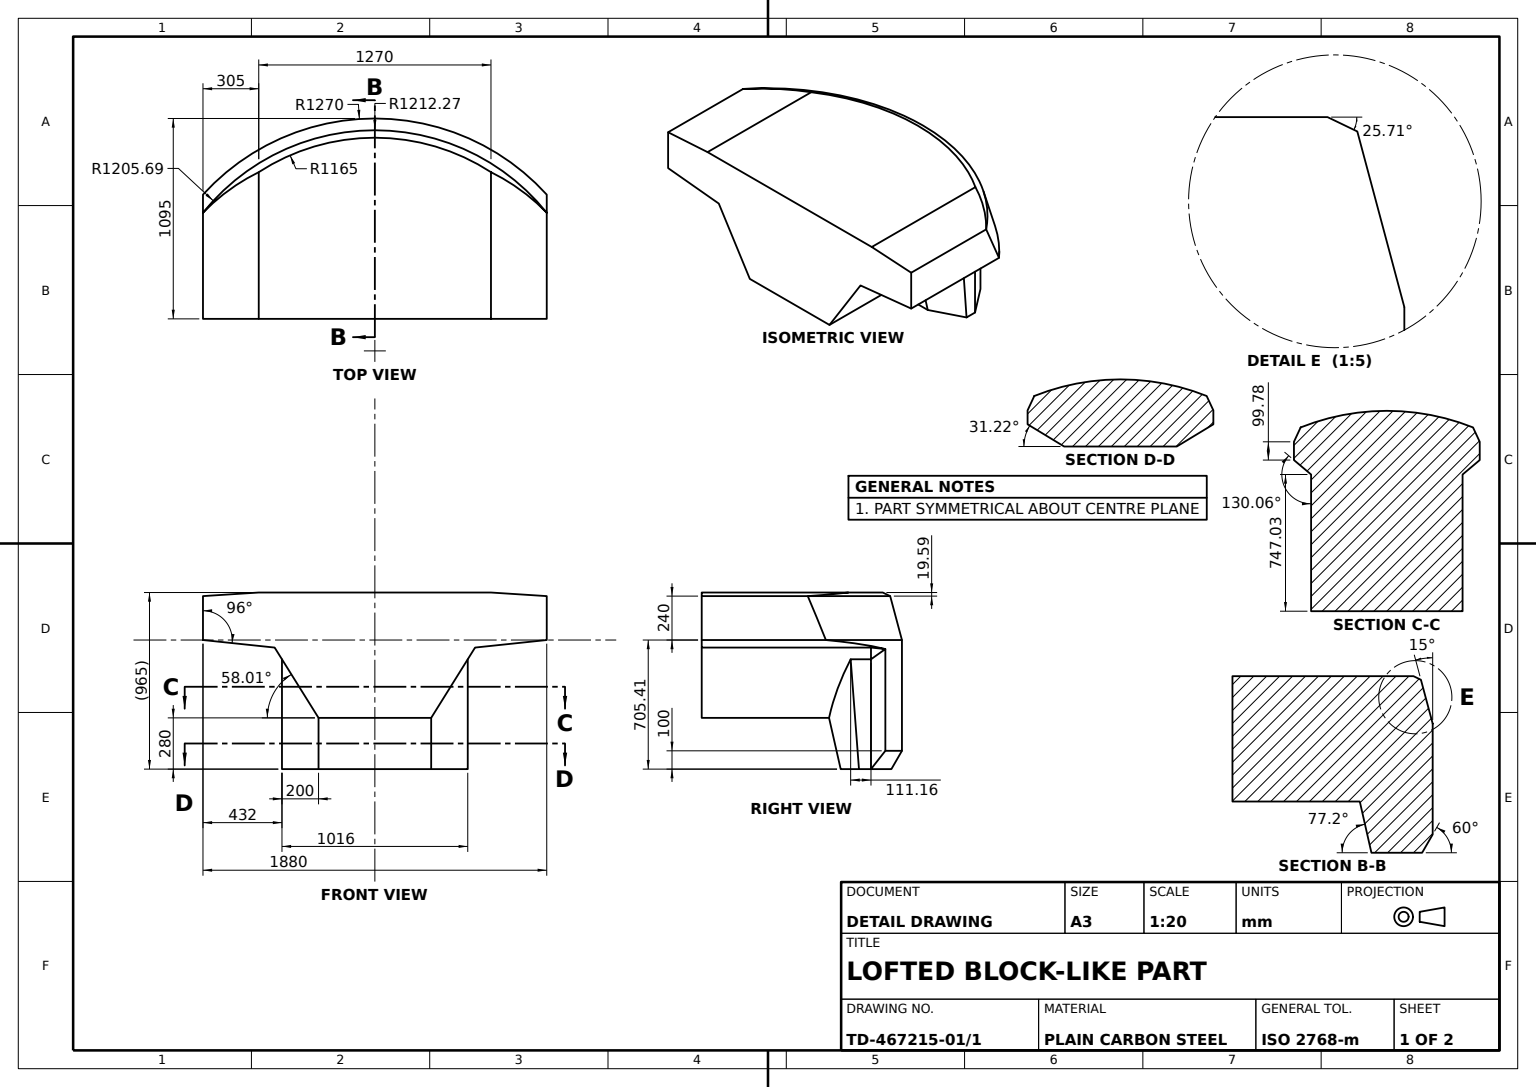
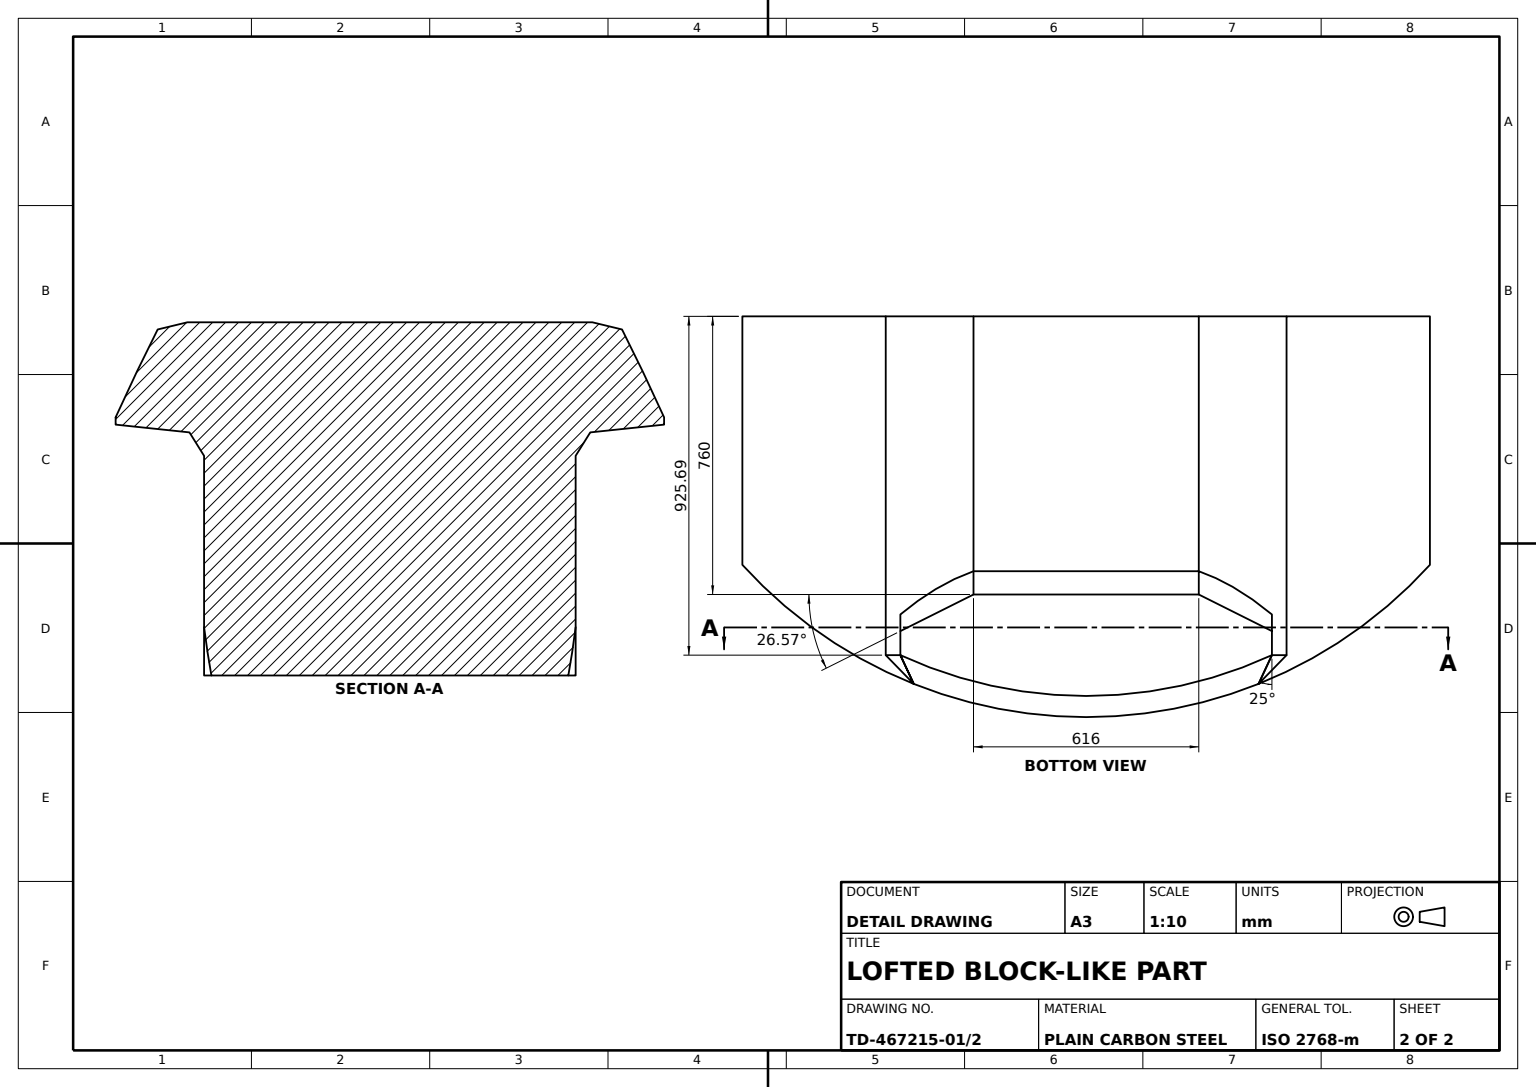
ISO-10303-21;
HEADER;
FILE_DESCRIPTION((''),'2;1');
FILE_NAME('','',(''),(''),'','','');
FILE_SCHEMA(('AUTOMOTIVE_DESIGN'));
ENDSEC;
DATA;
#1=APPLICATION_CONTEXT('');
#2=PRODUCT_CONTEXT('',#1,'mechanical');
#3=PRODUCT('','','',(#2));
#4=PRODUCT_DEFINITION_FORMATION('','',#3);
#5=PRODUCT_DEFINITION_CONTEXT('',#1,'design');
#6=PRODUCT_DEFINITION('','',#4,#5);
#7=PRODUCT_DEFINITION_SHAPE('','',#6);
#8=(LENGTH_UNIT()NAMED_UNIT(*)SI_UNIT(.MILLI.,.METRE.));
#9=(NAMED_UNIT(*)PLANE_ANGLE_UNIT()SI_UNIT($,.RADIAN.));
#10=(NAMED_UNIT(*)SI_UNIT($,.STERADIAN.)SOLID_ANGLE_UNIT());
#11=UNCERTAINTY_MEASURE_WITH_UNIT(LENGTH_MEASURE(1.E-05),#8,'distance_accuracy_value','');
#12=(GEOMETRIC_REPRESENTATION_CONTEXT(3)GLOBAL_UNCERTAINTY_ASSIGNED_CONTEXT((#11))GLOBAL_UNIT_ASSIGNED_CONTEXT((#8,#9,#10))REPRESENTATION_CONTEXT('',''));
#13=CARTESIAN_POINT('',(-471.347784,656.147697,-1004.292698));
#14=VERTEX_POINT('',#13);
#15=CARTESIAN_POINT('',(-548.,664.204169,-925.691767));
#16=VERTEX_POINT('',#15);
#17=DIRECTION('',(-0.696304067,0.073184506,0.714006075));
#18=VECTOR('',#17,1000.);
#19=LINE('',#13,#18);
#20=EDGE_CURVE('',#14,#16,#19,.T.);
#21=ORIENTED_EDGE('',*,*,#20,.F.);
#22=CARTESIAN_POINT('',(-508.,600.170141,-925.691767));
#23=VERTEX_POINT('',#22);
#24=DIRECTION('',(-0.355078158,-0.542297561,0.761467568));
#25=VECTOR('',#24,1000.);
#26=LINE('',#13,#25);
#27=EDGE_CURVE('',#14,#23,#26,.T.);
#28=ORIENTED_EDGE('',*,*,#27,.T.);
#29=DIRECTION('',(0.529796363,-0.848124881,0.));
#30=VECTOR('',#29,1000.);
#31=LINE('',#15,#30);
#32=EDGE_CURVE('',#16,#23,#31,.T.);
#33=ORIENTED_EDGE('',*,*,#32,.F.);
#34=EDGE_LOOP('',(#21,#28,#33));
#35=FACE_OUTER_BOUND('',#34,.T.);
#36=CARTESIAN_POINT('',(-439.803143,-274.730892,-400.739829));
#37=DIRECTION('',(-0.671086691,-0.419206294,-0.611480773));
#38=DIRECTION('',(-0.67351782,0.,0.739170985));
#39=AXIS2_PLACEMENT_3D('',#36,#37,#38);
#40=PLANE('',#39);
#41=ADVANCED_FACE('',(#35),#40,.T.);
#42=CARTESIAN_POINT('',(0.,945.40503,-1030.692194));
#43=VERTEX_POINT('',#42);
#44=CARTESIAN_POINT('',(940.,945.40503,-580.045473));
#45=VERTEX_POINT('',#44);
#46=CARTESIAN_POINT('',(0.,945.40503,175.));
#47=DIRECTION('',(0.,-1.,0.));
#48=DIRECTION('',(0.,0.,-1.));
#49=AXIS2_PLACEMENT_3D('',#46,#47,#48);
#50=CIRCLE('',#49,1205.692194);
#51=EDGE_CURVE('',#43,#45,#50,.T.);
#52=ORIENTED_EDGE('',*,*,#51,.T.);
#53=CARTESIAN_POINT('',(940.,705.40503,-678.990632));
#54=VERTEX_POINT('',#53);
#55=CARTESIAN_POINT('',(940.,745.612267,-662.96898));
#56=CARTESIAN_POINT('',(940.,785.727052,-646.738003));
#57=CARTESIAN_POINT('',(940.,865.739298,-613.78401));
#58=CARTESIAN_POINT('',(940.,905.636865,-597.061233));
#59=B_SPLINE_CURVE_WITH_KNOTS('',3,(#53,#55,#56,#57,#58,#44),.UNSPECIFIED.,.F.,.F.,(4,2,4),(0.754872471,0.884630392,1.014388313),.UNSPECIFIED.);
#60=EDGE_CURVE('',#54,#45,#59,.T.);
#61=ORIENTED_EDGE('',*,*,#60,.F.);
#62=CARTESIAN_POINT('',(0.,705.40503,-1095.));
#63=VERTEX_POINT('',#62);
#64=CARTESIAN_POINT('',(0.,705.40503,175.));
#65=AXIS2_PLACEMENT_3D('',#64,#47,#48);
#66=CIRCLE('',#65,1270.);
#67=EDGE_CURVE('',#63,#54,#66,.T.);
#68=ORIENTED_EDGE('',*,*,#67,.F.);
#69=DIRECTION('',(0.,-0.965925826,-0.258819045));
#70=VECTOR('',#69,1000.);
#71=LINE('',#42,#70);
#72=EDGE_CURVE('',#43,#63,#71,.T.);
#73=ORIENTED_EDGE('',*,*,#72,.F.);
#74=EDGE_LOOP('',(#52,#61,#68,#73));
#75=FACE_OUTER_BOUND('',#74,.T.);
#76=CONICAL_SURFACE('',#49,1205.692193817,0.261799388);
#77=ADVANCED_FACE('',(#75),#76,.T.);
#78=CARTESIAN_POINT('',(508.,600.170141,-925.691767));
#79=VERTEX_POINT('',#78);
#80=CARTESIAN_POINT('',(508.,0.,-925.691767));
#81=VERTEX_POINT('',#80);
#82=CARTESIAN_POINT('',(508.,745.039237,-925.691767));
#83=VECTOR('',#47,1000.);
#84=LINE('',#82,#83);
#85=EDGE_CURVE('',#79,#81,#84,.T.);
#86=ORIENTED_EDGE('',*,*,#85,.T.);
#87=CARTESIAN_POINT('',(471.347784,100.,-1004.292698));
#88=VERTEX_POINT('',#87);
#89=CARTESIAN_POINT('',(483.369243,66.264561,-978.512595));
#90=CARTESIAN_POINT('',(495.570346,32.897774,-952.347245));
#91=B_SPLINE_CURVE_WITH_KNOTS('',3,(#87,#89,#90,#80),.UNSPECIFIED.,.F.,.F.,(4,4),(0.000000262,0.132369032),.UNSPECIFIED.);
#92=EDGE_CURVE('',#88,#81,#91,.T.);
#93=ORIENTED_EDGE('',*,*,#92,.F.);
#94=CARTESIAN_POINT('',(471.347784,656.147697,-1004.292698));
#95=VERTEX_POINT('',#94);
#96=CARTESIAN_POINT('',(471.347784,745.039237,-1004.292698));
#97=LINE('',#96,#83);
#98=EDGE_CURVE('',#95,#88,#97,.T.);
#99=ORIENTED_EDGE('',*,*,#98,.F.);
#100=DIRECTION('',(0.355078158,-0.542297561,0.761467568));
#101=VECTOR('',#100,1000.);
#102=LINE('',#94,#101);
#103=EDGE_CURVE('',#95,#79,#102,.T.);
#104=ORIENTED_EDGE('',*,*,#103,.T.);
#105=EDGE_LOOP('',(#86,#93,#99,#104));
#106=FACE_OUTER_BOUND('',#105,.T.);
#107=DIRECTION('',(-0.906307787,0.,0.422618262));
#108=DIRECTION('',(0.422618262,0.,0.906307787));
#109=AXIS2_PLACEMENT_3D('',#82,#107,#108);
#110=PLANE('',#109);
#111=ADVANCED_FACE('',(#106),#110,.F.);
#112=CARTESIAN_POINT('',(548.,664.204169,-925.691767));
#113=VERTEX_POINT('',#112);
#114=CARTESIAN_POINT('',(548.,664.204169,0.));
#115=VERTEX_POINT('',#114);
#116=DIRECTION('',(0.,0.,1.));
#117=VECTOR('',#116,1000.);
#118=LINE('',#112,#117);
#119=EDGE_CURVE('',#113,#115,#118,.T.);
#120=ORIENTED_EDGE('',*,*,#119,.T.);
#121=CARTESIAN_POINT('',(308.,280.,0.));
#122=VERTEX_POINT('',#121);
#123=DIRECTION('',(0.529796363,0.848124881,0.));
#124=VECTOR('',#123,1000.);
#125=LINE('',#121,#124);
#126=EDGE_CURVE('',#122,#115,#125,.T.);
#127=ORIENTED_EDGE('',*,*,#126,.F.);
#128=CARTESIAN_POINT('',(308.,280.,-696.363636));
#129=VERTEX_POINT('',#128);
#130=CARTESIAN_POINT('',(308.,280.,-925.691767));
#131=LINE('',#130,#117);
#132=EDGE_CURVE('',#129,#122,#131,.T.);
#133=ORIENTED_EDGE('',*,*,#132,.F.);
#134=CARTESIAN_POINT('',(508.,600.170141,-814.532565));
#135=VERTEX_POINT('',#134);
#136=CARTESIAN_POINT('',(491.980272,574.524948,-801.181759));
#137=CARTESIAN_POINT('',(475.793634,548.612558,-788.625015));
#138=CARTESIAN_POINT('',(455.337931,515.86603,-773.98717));
#139=CARTESIAN_POINT('',(451.235664,509.298914,-771.112533));
#140=CARTESIAN_POINT('',(443.00851,496.128468,-765.470873));
#141=CARTESIAN_POINT('',(438.882887,489.523962,-762.703374));
#142=CARTESIAN_POINT('',(426.477598,469.664947,-754.56895));
#143=CARTESIAN_POINT('',(418.170441,456.366429,-749.370582));
#144=CARTESIAN_POINT('',(401.48017,429.647796,-739.435331));
#145=CARTESIAN_POINT('',(393.097056,416.227682,-734.698447));
#146=CARTESIAN_POINT('',(376.252748,389.26246,-725.699057));
#147=CARTESIAN_POINT('',(367.789964,375.714806,-721.436009));
#148=CARTESIAN_POINT('',(342.321315,334.943302,-709.396412));
#149=CARTESIAN_POINT('',(325.222915,307.571316,-702.362232));
#150=B_SPLINE_CURVE_WITH_KNOTS('',3,(#134,#136,#137,#138,#139,#140,#141,#142,#143,#144,#145,#146,#147,#148,#149,#128),.UNSPECIFIED.,.F.,.F.,(4,2,2,2,2,2,2,4),(0.,0.099089394,0.123861743,0.148634091,0.198178789,0.247723486,0.297268183,0.396357577),.UNSPECIFIED.);
#151=EDGE_CURVE('',#135,#129,#150,.T.);
#152=ORIENTED_EDGE('',*,*,#151,.F.);
#153=CARTESIAN_POINT('',(508.,600.170141,-1245.));
#154=LINE('',#153,#117);
#155=EDGE_CURVE('',#79,#135,#154,.T.);
#156=ORIENTED_EDGE('',*,*,#155,.F.);
#157=LINE('',#130,#124);
#158=EDGE_CURVE('',#79,#113,#157,.T.);
#159=ORIENTED_EDGE('',*,*,#158,.T.);
#160=EDGE_LOOP('',(#120,#127,#133,#152,#156,#159));
#161=FACE_OUTER_BOUND('',#160,.T.);
#162=DIRECTION('',(0.848124881,-0.529796363,0.));
#163=AXIS2_PLACEMENT_3D('',#130,#162,#123);
#164=PLANE('',#163);
#165=ADVANCED_FACE('',(#161),#164,.T.);
#166=ORIENTED_EDGE('',*,*,#155,.T.);
#167=CARTESIAN_POINT('',(508.,0.,-860.));
#168=VERTEX_POINT('',#167);
#169=DIRECTION('',(0.,0.997142688,0.075541113));
#170=VECTOR('',#169,1000.);
#171=LINE('',#167,#170);
#172=EDGE_CURVE('',#168,#135,#171,.T.);
#173=ORIENTED_EDGE('',*,*,#172,.F.);
#174=CARTESIAN_POINT('',(508.,0.,-1245.));
#175=LINE('',#174,#117);
#176=EDGE_CURVE('',#81,#168,#175,.T.);
#177=ORIENTED_EDGE('',*,*,#176,.F.);
#178=ORIENTED_EDGE('',*,*,#85,.F.);
#179=EDGE_LOOP('',(#166,#173,#177,#178));
#180=FACE_OUTER_BOUND('',#179,.T.);
#181=DIRECTION('',(-1.,0.,0.));
#182=AXIS2_PLACEMENT_3D('',#174,#181,#116);
#183=PLANE('',#182);
#184=ADVANCED_FACE('',(#180),#183,.F.);
#185=CARTESIAN_POINT('',(-308.,280.,-696.363636));
#186=VERTEX_POINT('',#185);
#187=CARTESIAN_POINT('',(-508.,600.170141,-814.532565));
#188=VERTEX_POINT('',#187);
#189=CARTESIAN_POINT('',(-325.223184,307.571746,-702.362325));
#190=CARTESIAN_POINT('',(-342.31947,334.940347,-709.395792));
#191=CARTESIAN_POINT('',(-363.53797,368.907998,-719.425934));
#192=CARTESIAN_POINT('',(-367.774075,375.689371,-721.493893));
#193=CARTESIAN_POINT('',(-376.231258,389.228058,-725.752355));
#194=CARTESIAN_POINT('',(-380.453182,395.986728,-727.943316));
#195=CARTESIAN_POINT('',(-393.089676,416.215868,-734.694309));
#196=CARTESIAN_POINT('',(-401.473914,429.637782,-739.431731));
#197=CARTESIAN_POINT('',(-418.164445,456.356829,-749.366888));
#198=CARTESIAN_POINT('',(-426.470737,469.653963,-754.564625));
#199=CARTESIAN_POINT('',(-443.007509,496.126866,-765.407806));
#200=CARTESIAN_POINT('',(-451.239205,509.304582,-771.054287));
#201=CARTESIAN_POINT('',(-475.791522,548.609176,-788.623275));
#202=CARTESIAN_POINT('',(-491.980008,574.524526,-801.181539));
#203=B_SPLINE_CURVE_WITH_KNOTS('',3,(#185,#189,#190,#191,#192,#193,#194,#195,#196,#197,#198,#199,#200,#201,#202,#187),.UNSPECIFIED.,.F.,.F.,(4,2,2,2,2,2,2,4),(0.,0.099073271,0.123841589,0.148609906,0.198146542,0.247683177,0.297219813,0.396293084),.UNSPECIFIED.);
#204=EDGE_CURVE('',#186,#188,#203,.T.);
#205=ORIENTED_EDGE('',*,*,#204,.T.);
#206=CARTESIAN_POINT('',(-508.,0.,-860.));
#207=VERTEX_POINT('',#206);
#208=CARTESIAN_POINT('',(-508.,330.,-835.));
#209=LINE('',#208,#170);
#210=EDGE_CURVE('',#207,#188,#209,.T.);
#211=ORIENTED_EDGE('',*,*,#210,.F.);
#212=CARTESIAN_POINT('',(-308.,0.,-760.));
#213=VERTEX_POINT('',#212);
#214=DIRECTION('',(0.894427191,0.,0.447213595));
#215=VECTOR('',#214,1000.);
#216=LINE('',#206,#215);
#217=EDGE_CURVE('',#207,#213,#216,.T.);
#218=ORIENTED_EDGE('',*,*,#217,.T.);
#219=CARTESIAN_POINT('',(-308.,330.,-685.));
#220=DIRECTION('',(0.,-0.975132856,-0.221621104));
#221=VECTOR('',#220,1000.);
#222=LINE('',#219,#221);
#223=EDGE_CURVE('',#186,#213,#222,.T.);
#224=ORIENTED_EDGE('',*,*,#223,.F.);
#225=EDGE_LOOP('',(#205,#211,#218,#224));
#226=FACE_OUTER_BOUND('',#225,.T.);
#227=CARTESIAN_POINT('',(-308.,660.,-610.));
#228=CARTESIAN_POINT('',(-341.333333,0.,-776.666667));
#229=CARTESIAN_POINT('',(-341.333333,660.,-643.333333));
#230=CARTESIAN_POINT('',(-374.666667,0.,-793.333333));
#231=CARTESIAN_POINT('',(-374.666667,660.,-676.666667));
#232=CARTESIAN_POINT('',(-441.333333,0.,-826.666667));
#233=CARTESIAN_POINT('',(-441.333333,660.,-743.333333));
#234=CARTESIAN_POINT('',(-474.666667,0.,-843.333333));
#235=CARTESIAN_POINT('',(-474.666667,660.,-776.666667));
#236=CARTESIAN_POINT('',(-508.,660.,-810.));
#237=B_SPLINE_SURFACE_WITH_KNOTS('',3,1,((#212,#227),(#228,#229),(#230,#231),(#232,#233),(#234,#235),(#206,#236)),.UNSPECIFIED.,.F.,.F.,.F.,(4,2,4),(2,2),(0.,0.5,1.),(0.,1.),.UNSPECIFIED.);
#238=ADVANCED_FACE('',(#226),#237,.F.);
#239=CARTESIAN_POINT('',(308.,0.,-760.));
#240=VERTEX_POINT('',#239);
#241=DIRECTION('',(0.894427191,0.,-0.447213595));
#242=VECTOR('',#241,1000.);
#243=LINE('',#167,#242);
#244=EDGE_CURVE('',#240,#168,#243,.T.);
#245=ORIENTED_EDGE('',*,*,#244,.T.);
#246=ORIENTED_EDGE('',*,*,#172,.T.);
#247=ORIENTED_EDGE('',*,*,#151,.T.);
#248=CARTESIAN_POINT('',(308.,330.,-685.));
#249=DIRECTION('',(0.,0.975132856,0.221621104));
#250=VECTOR('',#249,1000.);
#251=LINE('',#248,#250);
#252=EDGE_CURVE('',#240,#129,#251,.T.);
#253=ORIENTED_EDGE('',*,*,#252,.F.);
#254=EDGE_LOOP('',(#245,#246,#247,#253));
#255=FACE_OUTER_BOUND('',#254,.T.);
#256=CARTESIAN_POINT('',(508.,660.,-810.));
#257=CARTESIAN_POINT('',(474.666667,0.,-843.333333));
#258=CARTESIAN_POINT('',(474.666667,660.,-776.666667));
#259=CARTESIAN_POINT('',(441.333333,0.,-826.666667));
#260=CARTESIAN_POINT('',(441.333333,660.,-743.333333));
#261=CARTESIAN_POINT('',(374.666667,0.,-793.333333));
#262=CARTESIAN_POINT('',(374.666667,660.,-676.666667));
#263=CARTESIAN_POINT('',(341.333333,0.,-776.666667));
#264=CARTESIAN_POINT('',(341.333333,660.,-643.333333));
#265=CARTESIAN_POINT('',(308.,660.,-610.));
#266=B_SPLINE_SURFACE_WITH_KNOTS('',3,1,((#167,#256),(#257,#258),(#259,#260),(#261,#262),(#263,#264),(#239,#265)),.UNSPECIFIED.,.F.,.F.,.F.,(4,2,4),(2,2),(0.,0.5,1.),(0.,1.),.UNSPECIFIED.);
#267=ADVANCED_FACE('',(#255),#266,.F.);
#268=CARTESIAN_POINT('',(940.,945.40503,0.));
#269=VERTEX_POINT('',#268);
#270=CARTESIAN_POINT('',(940.,945.40503,-1245.));
#271=LINE('',#270,#117);
#272=EDGE_CURVE('',#45,#269,#271,.T.);
#273=ORIENTED_EDGE('',*,*,#272,.F.);
#274=CARTESIAN_POINT('',(635.,965.,-801.729236));
#275=VERTEX_POINT('',#274);
#276=CARTESIAN_POINT('',(851.792172,951.072012,-671.068148));
#277=CARTESIAN_POINT('',(749.105928,957.669173,-745.703797));
#278=(BOUNDED_CURVE()B_SPLINE_CURVE(3,(#44,#276,#277,#274),.UNSPECIFIED.,.F.,.T.)B_SPLINE_CURVE_WITH_KNOTS((4,4),(0.765207077,1.110816144),.UNSPECIFIED.)CURVE()GEOMETRIC_REPRESENTATION_ITEM()RATIONAL_B_SPLINE_CURVE((1.,0.990070943,0.990070943,1.))REPRESENTATION_ITEM(''));
#279=EDGE_CURVE('',#45,#275,#278,.T.);
#280=ORIENTED_EDGE('',*,*,#279,.T.);
#281=CARTESIAN_POINT('',(635.,965.,0.));
#282=VERTEX_POINT('',#281);
#283=CARTESIAN_POINT('',(635.,965.,-1245.));
#284=LINE('',#283,#117);
#285=EDGE_CURVE('',#275,#282,#284,.T.);
#286=ORIENTED_EDGE('',*,*,#285,.T.);
#287=DIRECTION('',(0.997942605,-0.064113625,0.));
#288=VECTOR('',#287,1000.);
#289=LINE('',#268,#288);
#290=EDGE_CURVE('',#282,#269,#289,.T.);
#291=ORIENTED_EDGE('',*,*,#290,.T.);
#292=EDGE_LOOP('',(#273,#280,#286,#291));
#293=FACE_OUTER_BOUND('',#292,.T.);
#294=DIRECTION('',(-0.064113625,-0.997942605,0.));
#295=AXIS2_PLACEMENT_3D('',#270,#294,#287);
#296=PLANE('',#295);
#297=ADVANCED_FACE('',(#293),#296,.F.);
#298=CARTESIAN_POINT('',(-1496.,0.,-760.));
#299=DIRECTION('',(1.,0.,0.));
#300=VECTOR('',#299,1000.);
#301=LINE('',#298,#300);
#302=EDGE_CURVE('',#213,#240,#301,.T.);
#303=ORIENTED_EDGE('',*,*,#302,.T.);
#304=ORIENTED_EDGE('',*,*,#252,.T.);
#305=CARTESIAN_POINT('',(-1496.,280.,-696.363636));
#306=VECTOR('',#181,1000.);
#307=LINE('',#305,#306);
#308=EDGE_CURVE('',#129,#186,#307,.T.);
#309=ORIENTED_EDGE('',*,*,#308,.T.);
#310=ORIENTED_EDGE('',*,*,#223,.T.);
#311=EDGE_LOOP('',(#303,#304,#309,#310));
#312=FACE_OUTER_BOUND('',#311,.T.);
#313=CARTESIAN_POINT('',(-1496.,660.,-610.));
#314=DIRECTION('',(0.,0.221621104,-0.975132856));
#315=AXIS2_PLACEMENT_3D('',#313,#314,#249);
#316=PLANE('',#315);
#317=ADVANCED_FACE('',(#312),#316,.F.);
#318=CARTESIAN_POINT('',(-508.,0.,-925.691767));
#319=VERTEX_POINT('',#318);
#320=CARTESIAN_POINT('',(-508.,745.039237,-925.691767));
#321=LINE('',#320,#83);
#322=EDGE_CURVE('',#23,#319,#321,.T.);
#323=ORIENTED_EDGE('',*,*,#322,.F.);
#324=ORIENTED_EDGE('',*,*,#27,.F.);
#325=CARTESIAN_POINT('',(-471.347784,100.,-1004.292698));
#326=VERTEX_POINT('',#325);
#327=CARTESIAN_POINT('',(-471.347784,745.039237,-1004.292698));
#328=LINE('',#327,#83);
#329=EDGE_CURVE('',#14,#326,#328,.T.);
#330=ORIENTED_EDGE('',*,*,#329,.T.);
#331=CARTESIAN_POINT('',(-495.570346,32.897774,-952.347245));
#332=CARTESIAN_POINT('',(-483.369243,66.264561,-978.512595));
#333=B_SPLINE_CURVE_WITH_KNOTS('',3,(#318,#331,#332,#325),.UNSPECIFIED.,.F.,.F.,(4,4),(0.000000268,0.132369038),.UNSPECIFIED.);
#334=EDGE_CURVE('',#319,#326,#333,.T.);
#335=ORIENTED_EDGE('',*,*,#334,.F.);
#336=EDGE_LOOP('',(#323,#324,#330,#335));
#337=FACE_OUTER_BOUND('',#336,.T.);
#338=DIRECTION('',(0.906307787,0.,0.422618262));
#339=DIRECTION('',(0.422618262,0.,-0.906307787));
#340=AXIS2_PLACEMENT_3D('',#320,#338,#339);
#341=PLANE('',#340);
#342=ADVANCED_FACE('',(#337),#341,.F.);
#343=ORIENTED_EDGE('',*,*,#204,.F.);
#344=CARTESIAN_POINT('',(-308.,280.,0.));
#345=VERTEX_POINT('',#344);
#346=CARTESIAN_POINT('',(-308.,280.,-925.691767));
#347=LINE('',#346,#117);
#348=EDGE_CURVE('',#186,#345,#347,.T.);
#349=ORIENTED_EDGE('',*,*,#348,.T.);
#350=CARTESIAN_POINT('',(-548.,664.204169,0.));
#351=VERTEX_POINT('',#350);
#352=LINE('',#350,#30);
#353=EDGE_CURVE('',#351,#345,#352,.T.);
#354=ORIENTED_EDGE('',*,*,#353,.F.);
#355=LINE('',#15,#117);
#356=EDGE_CURVE('',#16,#351,#355,.T.);
#357=ORIENTED_EDGE('',*,*,#356,.F.);
#358=ORIENTED_EDGE('',*,*,#32,.T.);
#359=CARTESIAN_POINT('',(-508.,600.170141,-1245.));
#360=LINE('',#359,#117);
#361=EDGE_CURVE('',#23,#188,#360,.T.);
#362=ORIENTED_EDGE('',*,*,#361,.T.);
#363=EDGE_LOOP('',(#343,#349,#354,#357,#358,#362));
#364=FACE_OUTER_BOUND('',#363,.T.);
#365=DIRECTION('',(-0.848124881,-0.529796363,0.));
#366=AXIS2_PLACEMENT_3D('',#15,#365,#29);
#367=PLANE('',#366);
#368=ADVANCED_FACE('',(#364),#367,.T.);
#369=ORIENTED_EDGE('',*,*,#176,.T.);
#370=ORIENTED_EDGE('',*,*,#244,.F.);
#371=ORIENTED_EDGE('',*,*,#302,.F.);
#372=ORIENTED_EDGE('',*,*,#217,.F.);
#373=CARTESIAN_POINT('',(-508.,0.,-1245.));
#374=LINE('',#373,#117);
#375=EDGE_CURVE('',#319,#207,#374,.T.);
#376=ORIENTED_EDGE('',*,*,#375,.F.);
#377=CARTESIAN_POINT('',(0.,0.,175.));
#378=AXIS2_PLACEMENT_3D('',#377,#47,#48);
#379=CIRCLE('',#378,1212.264973);
#380=EDGE_CURVE('',#319,#81,#379,.T.);
#381=ORIENTED_EDGE('',*,*,#380,.T.);
#382=EDGE_LOOP('',(#369,#370,#371,#372,#376,#381));
#383=FACE_OUTER_BOUND('',#382,.T.);
#384=CARTESIAN_POINT('',(0.,0.,-1245.));
#385=AXIS2_PLACEMENT_3D('',#384,#47,#299);
#386=PLANE('',#385);
#387=ADVANCED_FACE('',(#383),#386,.T.);
#388=CARTESIAN_POINT('',(-635.,965.,0.));
#389=VERTEX_POINT('',#388);
#390=CARTESIAN_POINT('',(-940.,945.40503,0.));
#391=VERTEX_POINT('',#390);
#392=DIRECTION('',(-0.997942605,-0.064113625,0.));
#393=VECTOR('',#392,1000.);
#394=LINE('',#390,#393);
#395=EDGE_CURVE('',#389,#391,#394,.T.);
#396=ORIENTED_EDGE('',*,*,#395,.F.);
#397=CARTESIAN_POINT('',(-635.,965.,-801.729236));
#398=VERTEX_POINT('',#397);
#399=CARTESIAN_POINT('',(-635.,965.,-1245.));
#400=LINE('',#399,#117);
#401=EDGE_CURVE('',#398,#389,#400,.T.);
#402=ORIENTED_EDGE('',*,*,#401,.F.);
#403=CARTESIAN_POINT('',(-940.,945.40503,-580.045473));
#404=VERTEX_POINT('',#403);
#405=CARTESIAN_POINT('',(-851.792172,951.072012,-671.068148));
#406=CARTESIAN_POINT('',(-749.105928,957.669173,-745.703797));
#407=(BOUNDED_CURVE()B_SPLINE_CURVE(3,(#403,#405,#406,#397),.UNSPECIFIED.,.F.,.F.)B_SPLINE_CURVE_WITH_KNOTS((4,4),(0.765207077,1.110816144),.UNSPECIFIED.)CURVE()GEOMETRIC_REPRESENTATION_ITEM()RATIONAL_B_SPLINE_CURVE((1.,0.990070943,0.990070943,1.))REPRESENTATION_ITEM(''));
#408=EDGE_CURVE('',#404,#398,#407,.T.);
#409=ORIENTED_EDGE('',*,*,#408,.F.);
#410=CARTESIAN_POINT('',(-940.,945.40503,-1245.));
#411=LINE('',#410,#117);
#412=EDGE_CURVE('',#404,#391,#411,.T.);
#413=ORIENTED_EDGE('',*,*,#412,.T.);
#414=EDGE_LOOP('',(#396,#402,#409,#413));
#415=FACE_OUTER_BOUND('',#414,.T.);
#416=DIRECTION('',(-0.064113625,0.997942605,0.));
#417=AXIS2_PLACEMENT_3D('',#410,#416,#392);
#418=PLANE('',#417);
#419=ADVANCED_FACE('',(#415),#418,.T.);
#420=EDGE_CURVE('',#404,#43,#50,.T.);
#421=ORIENTED_EDGE('',*,*,#420,.F.);
#422=ORIENTED_EDGE('',*,*,#408,.T.);
#423=CARTESIAN_POINT('',(0.,965.,-990.));
#424=VERTEX_POINT('',#423);
#425=CARTESIAN_POINT('',(0.,965.,175.));
#426=AXIS2_PLACEMENT_3D('',#425,#47,#48);
#427=CIRCLE('',#426,1165.);
#428=EDGE_CURVE('',#398,#424,#427,.T.);
#429=ORIENTED_EDGE('',*,*,#428,.T.);
#430=DIRECTION('',(0.,-0.433859343,-0.900980616));
#431=VECTOR('',#430,1000.);
#432=LINE('',#423,#431);
#433=EDGE_CURVE('',#424,#43,#432,.T.);
#434=ORIENTED_EDGE('',*,*,#433,.T.);
#435=EDGE_LOOP('',(#421,#422,#429,#434));
#436=FACE_OUTER_BOUND('',#435,.T.);
#437=CONICAL_SURFACE('',#426,1165.,1.122024454);
#438=ADVANCED_FACE('',(#436),#437,.T.);
#439=CARTESIAN_POINT('',(-940.,705.40503,-678.990632));
#440=VERTEX_POINT('',#439);
#441=CARTESIAN_POINT('',(-650.988178,675.028663,-932.492794));
#442=CARTESIAN_POINT('',(-809.912521,691.732285,-822.179826));
#443=(BOUNDED_CURVE()B_SPLINE_CURVE(3,(#13,#441,#442,#439),.UNSPECIFIED.,.F.,.T.)B_SPLINE_CURVE_WITH_KNOTS((4,4),(1.951032718,2.40410085),.UNSPECIFIED.)CURVE()GEOMETRIC_REPRESENTATION_ITEM()RATIONAL_B_SPLINE_CURVE((1.,0.982967134,0.982967134,1.))REPRESENTATION_ITEM(''));
#444=EDGE_CURVE('',#14,#440,#443,.T.);
#445=ORIENTED_EDGE('',*,*,#444,.F.);
#446=ORIENTED_EDGE('',*,*,#20,.T.);
#447=ORIENTED_EDGE('',*,*,#356,.T.);
#448=CARTESIAN_POINT('',(-940.,705.40503,0.));
#449=VERTEX_POINT('',#448);
#450=CARTESIAN_POINT('',(-508.,660.,0.));
#451=DIRECTION('',(0.994521895,-0.104528463,0.));
#452=VECTOR('',#451,1000.);
#453=LINE('',#450,#452);
#454=EDGE_CURVE('',#449,#351,#453,.T.);
#455=ORIENTED_EDGE('',*,*,#454,.F.);
#456=CARTESIAN_POINT('',(-940.,705.40503,-1245.));
#457=LINE('',#456,#117);
#458=EDGE_CURVE('',#440,#449,#457,.T.);
#459=ORIENTED_EDGE('',*,*,#458,.F.);
#460=EDGE_LOOP('',(#445,#446,#447,#455,#459));
#461=FACE_OUTER_BOUND('',#460,.T.);
#462=CARTESIAN_POINT('',(-508.,660.,-1245.));
#463=DIRECTION('',(-0.104528463,-0.994521895,0.));
#464=AXIS2_PLACEMENT_3D('',#462,#463,#451);
#465=PLANE('',#464);
#466=ADVANCED_FACE('',(#461),#465,.T.);
#467=ORIENTED_EDGE('',*,*,#444,.T.);
#468=EDGE_CURVE('',#440,#63,#66,.T.);
#469=ORIENTED_EDGE('',*,*,#468,.T.);
#470=CARTESIAN_POINT('',(0.,100.,-1095.));
#471=VERTEX_POINT('',#470);
#472=CARTESIAN_POINT('',(0.,2302.808193,-1095.));
#473=LINE('',#472,#83);
#474=EDGE_CURVE('',#63,#471,#473,.T.);
#475=ORIENTED_EDGE('',*,*,#474,.T.);
#476=CARTESIAN_POINT('',(0.,100.,175.));
#477=AXIS2_PLACEMENT_3D('',#476,#47,#48);
#478=CIRCLE('',#477,1270.);
#479=EDGE_CURVE('',#326,#471,#478,.T.);
#480=ORIENTED_EDGE('',*,*,#479,.F.);
#481=ORIENTED_EDGE('',*,*,#329,.F.);
#482=EDGE_LOOP('',(#467,#469,#475,#480,#481));
#483=FACE_OUTER_BOUND('',#482,.T.);
#484=CARTESIAN_POINT('',(0.,2302.808193,175.));
#485=AXIS2_PLACEMENT_3D('',#484,#47,#48);
#486=CYLINDRICAL_SURFACE('',#485,1270.);
#487=ADVANCED_FACE('',(#483),#486,.T.);
#488=ORIENTED_EDGE('',*,*,#92,.T.);
#489=ORIENTED_EDGE('',*,*,#380,.F.);
#490=ORIENTED_EDGE('',*,*,#334,.T.);
#491=ORIENTED_EDGE('',*,*,#479,.T.);
#492=EDGE_CURVE('',#471,#88,#478,.T.);
#493=ORIENTED_EDGE('',*,*,#492,.T.);
#494=EDGE_LOOP('',(#488,#489,#490,#491,#493));
#495=FACE_OUTER_BOUND('',#494,.T.);
#496=DIRECTION('',(0.,1.,0.));
#497=AXIS2_PLACEMENT_3D('',#476,#496,#116);
#498=CONICAL_SURFACE('',#497,1270.,0.523598776);
#499=ADVANCED_FACE('',(#495),#498,.T.);
#500=ORIENTED_EDGE('',*,*,#474,.F.);
#501=ORIENTED_EDGE('',*,*,#67,.T.);
#502=CARTESIAN_POINT('',(650.988178,675.028663,-932.492794));
#503=CARTESIAN_POINT('',(809.912521,691.732285,-822.179826));
#504=(BOUNDED_CURVE()B_SPLINE_CURVE(3,(#94,#502,#503,#53),.UNSPECIFIED.,.F.,.T.)B_SPLINE_CURVE_WITH_KNOTS((4,4),(1.951032718,2.40410085),.UNSPECIFIED.)CURVE()GEOMETRIC_REPRESENTATION_ITEM()RATIONAL_B_SPLINE_CURVE((1.,0.982967134,0.982967134,1.))REPRESENTATION_ITEM(''));
#505=EDGE_CURVE('',#95,#54,#504,.T.);
#506=ORIENTED_EDGE('',*,*,#505,.F.);
#507=ORIENTED_EDGE('',*,*,#98,.T.);
#508=ORIENTED_EDGE('',*,*,#492,.F.);
#509=EDGE_LOOP('',(#500,#501,#506,#507,#508));
#510=FACE_OUTER_BOUND('',#509,.T.);
#511=ADVANCED_FACE('',(#510),#486,.T.);
#512=ORIENTED_EDGE('',*,*,#60,.T.);
#513=ORIENTED_EDGE('',*,*,#272,.T.);
#514=CARTESIAN_POINT('',(940.,705.40503,0.));
#515=VERTEX_POINT('',#514);
#516=LINE('',#514,#83);
#517=EDGE_CURVE('',#269,#515,#516,.T.);
#518=ORIENTED_EDGE('',*,*,#517,.T.);
#519=CARTESIAN_POINT('',(940.,705.40503,-1245.));
#520=LINE('',#519,#117);
#521=EDGE_CURVE('',#54,#515,#520,.T.);
#522=ORIENTED_EDGE('',*,*,#521,.F.);
#523=EDGE_LOOP('',(#512,#513,#518,#522));
#524=FACE_OUTER_BOUND('',#523,.T.);
#525=AXIS2_PLACEMENT_3D('',#519,#181,#116);
#526=PLANE('',#525);
#527=ADVANCED_FACE('',(#524),#526,.F.);
#528=ORIENTED_EDGE('',*,*,#308,.F.);
#529=ORIENTED_EDGE('',*,*,#132,.T.);
#530=LINE('',#344,#300);
#531=EDGE_CURVE('',#345,#122,#530,.T.);
#532=ORIENTED_EDGE('',*,*,#531,.F.);
#533=ORIENTED_EDGE('',*,*,#348,.F.);
#534=EDGE_LOOP('',(#528,#529,#532,#533));
#535=FACE_OUTER_BOUND('',#534,.T.);
#536=AXIS2_PLACEMENT_3D('',#346,#47,#48);
#537=PLANE('',#536);
#538=ADVANCED_FACE('',(#535),#537,.T.);
#539=DIRECTION('',(0.696304067,0.073184506,0.714006075));
#540=VECTOR('',#539,1000.);
#541=LINE('',#94,#540);
#542=EDGE_CURVE('',#95,#113,#541,.T.);
#543=ORIENTED_EDGE('',*,*,#542,.T.);
#544=ORIENTED_EDGE('',*,*,#158,.F.);
#545=ORIENTED_EDGE('',*,*,#103,.F.);
#546=EDGE_LOOP('',(#543,#544,#545));
#547=FACE_OUTER_BOUND('',#546,.T.);
#548=CARTESIAN_POINT('',(439.803143,-274.730892,-400.739829));
#549=DIRECTION('',(-0.671086691,0.419206294,0.611480773));
#550=DIRECTION('',(0.67351782,0.,0.739170985));
#551=AXIS2_PLACEMENT_3D('',#548,#549,#550);
#552=PLANE('',#551);
#553=ADVANCED_FACE('',(#547),#552,.F.);
#554=ORIENTED_EDGE('',*,*,#395,.T.);
#555=LINE('',#448,#83);
#556=EDGE_CURVE('',#391,#449,#555,.T.);
#557=ORIENTED_EDGE('',*,*,#556,.T.);
#558=ORIENTED_EDGE('',*,*,#454,.T.);
#559=ORIENTED_EDGE('',*,*,#353,.T.);
#560=ORIENTED_EDGE('',*,*,#531,.T.);
#561=ORIENTED_EDGE('',*,*,#126,.T.);
#562=CARTESIAN_POINT('',(508.,660.,0.));
#563=DIRECTION('',(-0.994521895,-0.104528463,0.));
#564=VECTOR('',#563,1000.);
#565=LINE('',#562,#564);
#566=EDGE_CURVE('',#515,#115,#565,.T.);
#567=ORIENTED_EDGE('',*,*,#566,.F.);
#568=ORIENTED_EDGE('',*,*,#517,.F.);
#569=ORIENTED_EDGE('',*,*,#290,.F.);
#570=LINE('',#388,#306);
#571=EDGE_CURVE('',#282,#389,#570,.T.);
#572=ORIENTED_EDGE('',*,*,#571,.T.);
#573=EDGE_LOOP('',(#554,#557,#558,#559,#560,#561,#567,#568,#569,#572));
#574=FACE_OUTER_BOUND('',#573,.T.);
#575=CARTESIAN_POINT('',(0.,0.,0.));
#576=AXIS2_PLACEMENT_3D('',#575,#48,#181);
#577=PLANE('',#576);
#578=ADVANCED_FACE('',(#574),#577,.F.);
#579=ORIENTED_EDGE('',*,*,#119,.F.);
#580=ORIENTED_EDGE('',*,*,#542,.F.);
#581=ORIENTED_EDGE('',*,*,#505,.T.);
#582=ORIENTED_EDGE('',*,*,#521,.T.);
#583=ORIENTED_EDGE('',*,*,#566,.T.);
#584=EDGE_LOOP('',(#579,#580,#581,#582,#583));
#585=FACE_OUTER_BOUND('',#584,.T.);
#586=CARTESIAN_POINT('',(508.,660.,-1245.));
#587=DIRECTION('',(-0.104528463,0.994521895,0.));
#588=AXIS2_PLACEMENT_3D('',#586,#587,#563);
#589=PLANE('',#588);
#590=ADVANCED_FACE('',(#585),#589,.F.);
#591=ORIENTED_EDGE('',*,*,#412,.F.);
#592=CARTESIAN_POINT('',(-940.,745.612267,-662.96898));
#593=CARTESIAN_POINT('',(-940.,785.727052,-646.738003));
#594=CARTESIAN_POINT('',(-940.,865.739298,-613.78401));
#595=CARTESIAN_POINT('',(-940.,905.636865,-597.061233));
#596=B_SPLINE_CURVE_WITH_KNOTS('',3,(#439,#592,#593,#594,#595,#403),.UNSPECIFIED.,.F.,.F.,(4,2,4),(0.754872471,0.884630392,1.014388313),.UNSPECIFIED.);
#597=EDGE_CURVE('',#440,#404,#596,.T.);
#598=ORIENTED_EDGE('',*,*,#597,.F.);
#599=ORIENTED_EDGE('',*,*,#458,.T.);
#600=ORIENTED_EDGE('',*,*,#556,.F.);
#601=EDGE_LOOP('',(#591,#598,#599,#600));
#602=FACE_OUTER_BOUND('',#601,.T.);
#603=AXIS2_PLACEMENT_3D('',#456,#181,#116);
#604=PLANE('',#603);
#605=ADVANCED_FACE('',(#602),#604,.T.);
#606=ORIENTED_EDGE('',*,*,#571,.F.);
#607=ORIENTED_EDGE('',*,*,#285,.F.);
#608=EDGE_CURVE('',#424,#275,#427,.T.);
#609=ORIENTED_EDGE('',*,*,#608,.F.);
#610=ORIENTED_EDGE('',*,*,#428,.F.);
#611=ORIENTED_EDGE('',*,*,#401,.T.);
#612=EDGE_LOOP('',(#606,#607,#609,#610,#611));
#613=FACE_OUTER_BOUND('',#612,.T.);
#614=AXIS2_PLACEMENT_3D('',#399,#496,#181);
#615=PLANE('',#614);
#616=ADVANCED_FACE('',(#613),#615,.T.);
#617=ORIENTED_EDGE('',*,*,#322,.T.);
#618=ORIENTED_EDGE('',*,*,#375,.T.);
#619=ORIENTED_EDGE('',*,*,#210,.T.);
#620=ORIENTED_EDGE('',*,*,#361,.F.);
#621=EDGE_LOOP('',(#617,#618,#619,#620));
#622=FACE_OUTER_BOUND('',#621,.T.);
#623=AXIS2_PLACEMENT_3D('',#373,#181,#116);
#624=PLANE('',#623);
#625=ADVANCED_FACE('',(#622),#624,.T.);
#626=ORIENTED_EDGE('',*,*,#279,.F.);
#627=ORIENTED_EDGE('',*,*,#51,.F.);
#628=ORIENTED_EDGE('',*,*,#433,.F.);
#629=ORIENTED_EDGE('',*,*,#608,.T.);
#630=EDGE_LOOP('',(#626,#627,#628,#629));
#631=FACE_OUTER_BOUND('',#630,.T.);
#632=ADVANCED_FACE('',(#631),#437,.T.);
#633=ORIENTED_EDGE('',*,*,#597,.T.);
#634=ORIENTED_EDGE('',*,*,#420,.T.);
#635=ORIENTED_EDGE('',*,*,#72,.T.);
#636=ORIENTED_EDGE('',*,*,#468,.F.);
#637=EDGE_LOOP('',(#633,#634,#635,#636));
#638=FACE_OUTER_BOUND('',#637,.T.);
#639=ADVANCED_FACE('',(#638),#76,.T.);
#640=CLOSED_SHELL('',(#41,#77,#111,#165,#184,#238,#267,#297,#317,#342,#368,#387,#419,#438,#466,#487,#499,#511,#527,#538,#553,#578,#590,#605,#616,#625,#632,#639));
#641=MANIFOLD_SOLID_BREP('',#640);
#642=ADVANCED_BREP_SHAPE_REPRESENTATION('',(#641),#12);
#643=SHAPE_DEFINITION_REPRESENTATION(#7,#642);
ENDSEC;
END-ISO-10303-21;
